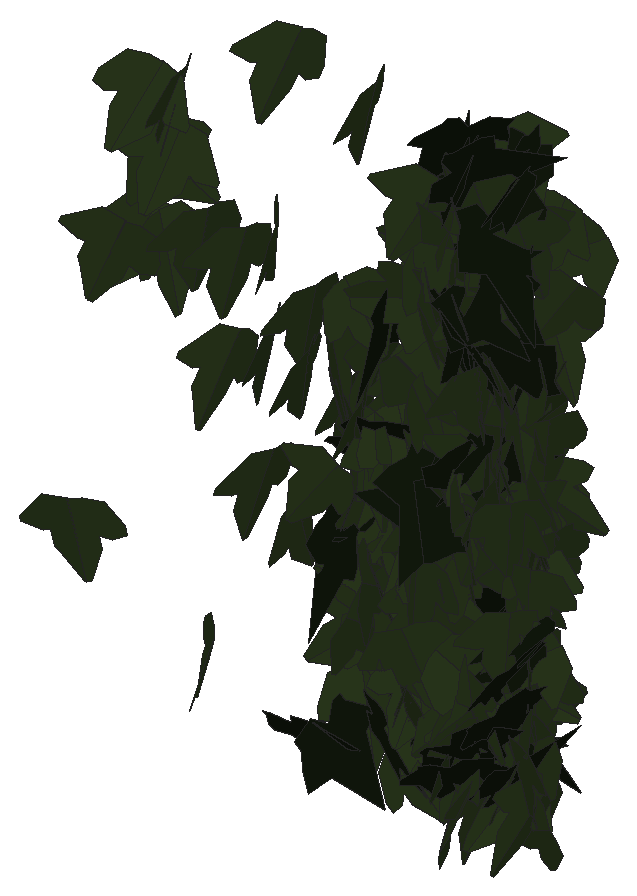
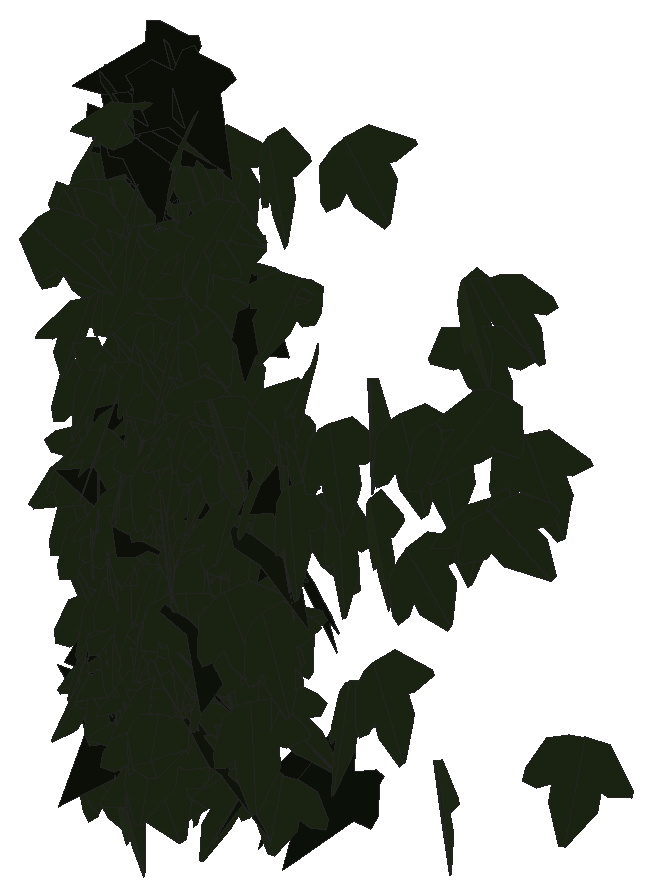
# SketchUp Ruby script. Lengths in inches.
U = 1.inch
M = Sketchup.active_model
def pt(a) = Geom::Point3d.new(a.map { |v| v * U })
def face(e, loops, mat)
  f = e.add_face(loops[0].map { |a| pt(a) })
  loops[1..].each { |l| e.add_face(l.map { |a| pt(a) }).erase! }
  f.material = f.back_material = mat if mat
  f
end
# faces: each face lists its corners as indices into pts; further lists are holes
def faces(e, pts, list, mat = nil) = list.each { |f| face(e, (f[0].is_a?(Array) ? f : [f]).map { |l| l.map { |i| pts[i] } }, mat) }
# xy, xz, yz: faces in a plane at the given z, y or x. An outline is a flat list of corners, or four numbers for a rectangle; further outlines are holes
def ring(l) = l.size == 4 ? [[l[0], l[1]], [l[2], l[1]], [l[2], l[3]], [l[0], l[3]]] : l.each_slice(2).to_a
def flat(e, list, mat, &to3) = list.each { |f| face(e, (f[0].is_a?(Array) ? f : [f]).map { |l| ring(l).map { |u, v| to3.(u, v) } }, mat) }
def xy(e, z, list, mat = nil) = flat(e, list, mat) { |x, y| [x, y, z] }
def xz(e, y, list, mat = nil) = flat(e, list, mat) { |x, z| [x, y, z] }
def yz(e, x, list, mat = nil) = flat(e, list, mat) { |y, z| [x, y, z] }
def lines(e, pts, list) = list.each { |a, b| e.add_line(pt(pts[a]), pt(pts[b])) }
# prism: a flat outline (further loops are holes) pulled along v
def prism(e, loops, v, mat = nil)
  f = face(e, loops, mat); d = Geom::Vector3d.new(v.map { |x| x * U })
  f.pushpull(f.normal.samedirection?(d) ? d.length : -d.length)
end
def box(e, o, s, mat = nil) = prism(e, [[o, [o[0] + s[0], o[1], o[2]], [o[0] + s[0], o[1] + s[1], o[2]], [o[0], o[1] + s[1], o[2]]]], [0, 0, s[2]], mat)
def at(x, y, z, deg = 0) = Geom::Transformation.translation(pt([x, y, z])) * Geom::Transformation.rotation(ORIGIN, Z_AXIS, deg.degrees)
def axes(o, x, y, z) = Geom::Transformation.new([*x, 0, *y, 0, *z, 0, *pt(o).to_a, 1])
def part(name) = M.definitions.add(name)
# library, detail: a bought-in or finely detailed component or shape, given as its bounding box
def library(name, o, s) = part(name).tap { |d| box(d.entities, o, s) }
def detail(e, o, s) = box(e.add_group.entities, o, s)
def put(e, d, t, mat = nil) = e.add_instance(d, t).tap { |i| i.material = mat if mat }
def group(e, t, mat = nil) = e.add_group.tap { |g| g.transformation = t; g.material = mat if mat }.entities
root = M.entities
M.materials.add("efeu1").color = [18, 25, 13]
M.materials.add("efeu2").color = [43, 57, 29]
c1 = part("ivyleaf_10")
p = [[0,0.5,-0.03],[-0.0625,2.02,-0.43],[-0.19,2.01,-0.46],[-0.54,1.05,-0.29],[-0.52,0.625,-0.18],[-0.83,0.76,-0.28],
  [-1.16,0.64,-0.33],[-1.15,0.33,-0.24],[-0.77,-0.39,0.02],[-0.3,-0.51,0.16],[0.04,-0.48,0.23],[-0.02,2.01,-0.4375],
  [-0.06,2.01,-0.43],[0.04,-0.49,0.23],[0.67,-0.49,0.14],[1.38,0.36,-0.2],[1.375,0.51,-0.24],[0.81,0.65,-0.19],
  [0.62,0.59,-0.15],[0.6,1.09,-0.28],[0.5,1.23,-0.31]]
faces(c1.entities,p,[[0,1,2,3,4,5,6,7,8,9,10],[11,12,0,13,14,15,16,17,18,19,20]],"efeu2")
c2 = part("ivyleaf_9")
p = [[1.54,2.16,1.25],[1.36,2.04,1.19],[-0.21,0.99,0.68],[-0.71,1.11,0.82],[-0.85,0.86,0.67],[-0.8,0.17,0.21],
  [-0.9,-0.01,0.1],[-0.67,-0.16,-0.02],[-0.08,-0.08,-0.05],[-0.03,-0.6,-0.4],[0.65,-0.88,-0.66],[0.83,-0.6,-0.49],
  [1.29,-0.42,-0.43],[1.8125,-0.07,-0.26],[1.21,0.44,0.15]]
faces(c2.entities,p,[[0,1,2,3,4,5,6,7,8,9,10,11,12,13,14]],"efeu1")
put(root,c1,axes([0.96,224.34,216.06],[-0.47039,-0.16713,-0.02836],[0.02619,0.01099,-0.49919],[0.16749,-0.47111,-0.00158]))
put(root,c1,axes([1.1875,225.43,219.52],[0.31206,0.2858,-0.26634],[-0.22229,-0.15043,-0.42185],[-0.32126,0.38169,0.03318]))
put(root,c1,axes([1.51,224.51,219.83],[-0.41225,-0.19131,0.20845],[-0.16107,-0.14417,-0.45086],[0.23261,-0.43888,0.05723]))
put(root,c1,axes([1.5,225.36,219.49],[0.05579,0.49599,0.02976],[-0.00377,0.03037,-0.49906],[-0.49686,0.05546,0.00713]))
put(root,c1,axes([1.57,225.19,220.67],[-0.1581,-0.36154,-0.30707],[0.26894,0.19831,-0.37195],[0.39074,-0.28278,0.13176]))
put(root,c1,axes([1.82,224.67,221.91],[0.46103,0.07291,-0.17927],[-0.17636,-0.03246,-0.46674],[-0.0797,0.49359,-0.00422]))
put(root,c1,axes([2.03,224.92,221.83],[0.1465,-0.47798,0.00877],[0.00356,-0.00808,-0.49992],[0.47804,0.14654,0.00103]))
put(root,c1,axes([2.11,224.74,221.18],[0.46588,0.12341,-0.13313],[-0.1388,0.00583,-0.48031],[-0.117,0.4845,0.03969]))
put(root,c1,axes([2.26,225.125,220],[-0.16365,-0.472,0.02088],[-0.00643,-0.01987,-0.49956],[0.47242,-0.16378,0.00044]))
put(root,c1,axes([2.54,225.25,218.39],[-0.09392,-0.42921,0.23866],[0.04424,-0.24939,-0.4311],[0.4891,-0.05986,0.08482]))
put(root,c1,axes([2.8,225.11,219.92],[-0.14469,-0.46928,0.09402],[0.00852,-0.10073,-0.48967],[0.47853,-0.1401,0.03714]))
put(root,c1,axes([2.88,225.47,216.86],[-0.04373,-0.49068,0.08555],[0.00052,-0.08593,-0.49256],[0.49808,-0.04299,0.00802]))
put(root,c1,axes([3,224.25,215.01],[0.21326,-0.39005,-0.22888],[-0.0988,0.20675,-0.4444],[0.44132,0.23477,0.01111]))
put(root,c1,axes([3.13,225.24,218.76],[0.17755,-0.46436,-0.05333],[-0.00564,0.05491,-0.49694],[0.46738,0.17706,0.01426]))
put(root,c1,axes([3.26,225.14,220.21],[0.19492,-0.39777,-0.23192],[-0.05057,0.23182,-0.44011],[0.45766,0.19503,0.05014]))
put(root,c1,axes([3.33,225.48,216.4375],[0.09135,-0.45267,-0.1917],[0.0624,0.20408,-0.45217],[0.48761,0.05869,0.09378]))
put(root,c1,axes([3.6,225.28,218.55],[0.07334,-0.47095,-0.15108],[-0.02799,0.14853,-0.47661],[0.4938,0.07837,-0.00458]))
put(root,c1,axes([3.77,225.21,219.48],[-0.06818,-0.49522,-0.01044],[0.00123,0.01037,-0.49989],[0.49533,-0.06819,-0.00019]))
put(root,c1,axes([3.8,224.81,223.01],[-0.21603,-0.39611,0.21548],[-0.0125,-0.23357,-0.44191],[0.45075,-0.19632,0.09101]))
put(root,c1,axes([4.31,225.27,218.5],[0.0717,-0.48644,-0.09072],[0.00628,0.09256,-0.49132],[0.49479,0.06932,0.01938]))
put(root,c1,axes([4.5,225.4375,216.91],[-0.03153,-0.49581,0.05635],[-0.00224,-0.05632,-0.49681],[0.499,-0.03159,0.00133]))
put(root,c1,axes([4.71,224.38,217.85],[-0.36088,-0.07697,0.27837],[-0.2598,-0.13092,-0.35148],[0.15159,-0.40763,0.06032]))
put(root,c2,axes([4.4,224.12,214.57],[0.43898,0.13994,-0.06919],[-0.09411,0.05199,-0.43992],[-0.13838,0.40858,0.07967]))
put(root,c1,axes([4.8125,224.95,215.67],[0.34304,-0.0201,-0.3632],[-0.36196,0.03072,-0.34357],[0.03613,0.49865,0.00653]))
put(root,c1,axes([4.66,225.55,215.74],[-0.16669,-0.47025,-0.03289],[0.00787,0.03211,-0.49891],[0.47133,-0.16685,-0.0033]))
put(root,c1,axes([4.87,224.73,217.83],[0.19361,-0.39179,-0.24293],[-0.11098,0.21612,-0.43701],[0.44743,0.22314,-0.00327]))
put(root,c1,axes([4.61,225.07,214.73],[0.46794,0.10225,0.14346],[0.13534,0.05202,-0.47852],[-0.11279,0.48666,0.02101]))
put(root,c1,axes([4.94,225.1875,216.31],[-0.47803,-0.05598,0.13549],[-0.13614,-0.00191,-0.4811],[0.05438,-0.49685,-0.01342]))
put(root,c1,axes([4.78,224.46,218.87],[-0.34673,0.29272,-0.02245],[0.00861,-0.02329,-0.45168],[-0.31688,-0.32093,0.0123]))
put(root,c1,axes([4.86,224.91,222.66],[0.10278,-0.48698,-0.04785],[-0.00495,0.04785,-0.49768],[0.4893,0.10278,0.00502]))
put(root,c2,axes([4.87,224.38,217.11],[-0.37707,0.05574,-0.26356],[0.27267,-0.02508,-0.36748],[-0.06468,-0.43068,-0.01271]))
put(root,c1,axes([4.83,224.33,219.67],[-0.15891,0.40661,-0.04926],[0.00632,-0.04824,-0.44957],[-0.44206,-0.14685,0.01128]))
put(root,c2,axes([5.2,224.65,217.49],[-0.13651,0.37995,0.17676],[-0.17867,0.11713,-0.40028],[-0.4125,-0.17647,0.11488]))
put(root,c1,axes([5.0625,225.41,216.97],[-0.20223,-0.4241,0.17101],[-0.00333,-0.18562,-0.46426],[0.45727,-0.18891,0.07225]))
put(root,c2,axes([4.9,224.15,214.7],[0.10876,-0.25337,-0.35251],[-0.14432,0.31155,-0.28349],[0.43365,0.16723,-0.00594]))
put(root,c1,axes([4.97,225,219.26],[0.0369,-0.36666,0.33793],[0.12839,-0.32044,-0.36171],[0.48182,0.11347,0.0705]))
put(root,c1,axes([5.08,224.52,218.6],[-0.43364,0.16052,-0.04923],[-0.02147,-0.16793,-0.41682],[-0.17946,-0.36777,0.16883]))
put(root,c1,axes([5.17,224.33,218.92],[0.0818,-0.37126,-0.22221],[-0.04888,0.20883,-0.39406],[0.46003,0.0882,-0.00236]))
put(root,c1,axes([4.83,225.12,216.41],[0.35816,-0.09659,0.33525],[0.32701,-0.07452,-0.37083],[0.1216,0.48489,0.00979]))
put(root,c1,axes([5.4,224.52,216.24],[0.1932,0.12468,0.39146],[-0.34982,-0.19223,0.22632],[0.247,-0.36977,0.01434]))
put(root,c1,axes([5.04,225.17,216.64],[-0.44515,0.05357,-0.22129],[0.21516,-0.05996,-0.44734],[-0.07447,-0.49349,0.03033]))
put(root,c1,axes([5.26,224.81,217.61],[-0.2177,-0.44259,-0.082],[0.04095,0.07124,-0.4932],[0.44825,-0.22146,0.00523]))
put(root,c1,axes([5.33,224.4375,216.76],[-0.3028,0.27586,0.19322],[-0.14349,0.12987,-0.40906],[-0.32929,-0.31026,0.00057]))
put(root,c2,axes([5.02,224.45,218.44],[0.40584,0.12435,0.18764],[0.17225,0.09041,-0.41026],[-0.16229,0.40692,0.03381]))
put(root,c1,axes([5.24,224.19,216.22],[-0.07236,-0.29876,-0.39434],[0.12552,0.37441,-0.30669],[0.47855,-0.14338,0.02082]))
put(root,c1,axes([5.24,225.3,218.19],[-0.02706,0.49926,0.00329],[-0.00013,0.00329,-0.49999],[-0.49927,-0.02706,-0.00005]))
put(root,c1,axes([5.17,224.74,218.29],[-0.01169,-0.46038,0.19472],[0.25019,-0.17402,-0.39639],[0.43275,0.08816,0.23443]))
put(root,c1,axes([5.22,224.17,220.49],[0.21395,0.33695,0.19854],[0.03353,0.19993,-0.40049],[-0.41691,0.18899,0.06968]))
put(root,c1,axes([5.3,225.09,218.53],[0.31704,-0.38619,0.01861],[0.00301,0.02653,0.49929],[-0.38663,-0.31647,0.01915]))
put(root,c1,axes([5.4375,224.11,216.8],[0.16934,-0.22854,-0.41121],[-0.00934,0.43532,-0.24579],[0.47036,0.09092,0.14316]))
put(root,c2,axes([5.31,224.47,214.8],[0.372,-0.13798,-0.23611],[-0.21395,0.11429,-0.38483],[0.19118,0.39639,0.02876]))
put(root,c1,axes([5.47,225.1875,218.97],[-0.19538,-0.45916,0.03151],[0.03111,-0.04733,-0.49678],[0.45919,-0.19217,0.04707]))
put(root,c2,axes([5.7,225.125,215.02],[-0.35311,0.28481,0.03615],[-0.03083,0.02015,-0.45094],[-0.30834,-0.32818,0.00369]))
put(root,c1,axes([5.5,225.19,219.11],[-0.25973,-0.42384,0.05387],[0.01978,-0.0749,-0.49396],[0.42679,-0.25446,0.05567]))
put(root,c1,axes([5.5,225.07,216.81],[-0.49206,0.07211,-0.05173],[0.05092,-0.00934,-0.49731],[-0.07269,-0.49468,0.00185]))
put(root,c2,axes([5.625,224.55,217.23],[0.2706,0.05186,-0.36586],[-0.38344,0.01246,-0.26107],[-0.02144,0.43172,0.05148]))
put(root,c1,axes([5.65,224.76,215.72],[0.34046,-0.21633,-0.29544],[-0.19484,0.23454,-0.39627],[0.31004,0.38496,0.0754]))
put(root,c1,axes([5.52,225.2,219.25],[0.38803,0.30743,-0.07012],[-0.09449,0.0073,-0.49094],[-0.30083,0.39425,0.06377]))
put(root,c1,axes([5.6,224.78,215.54],[0.26224,-0.41911,-0.07469],[-0.05121,0.05604,-0.4942],[0.42262,0.26685,-0.01353]))
put(root,c2,axes([5.5,224.55,220.36],[-0.12922,0.11287,-0.41881],[0.32083,-0.2719,-0.17105],[-0.31794,-0.32024,-0.00238]))
put(root,c1,axes([5.57,224.97,218.71],[-0.092,0.41612,0.26149],[-0.06876,0.25252,-0.42604],[-0.48663,-0.11435,0.01076]))
put(root,c1,axes([5.72,224.52,215.29],[-0.39409,0.21502,0.22013],[-0.186,0.11851,-0.44873],[-0.24515,-0.43557,-0.01342]))
put(root,c2,axes([5.69,224.84,216.53],[0.0985,0.41342,0.10395],[-0.0361,0.10888,-0.43662],[-0.45794,0.08034,0.05678]))
put(root,c1,axes([5.48,224.67,217.5],[0.40548,0.20234,0.08901],[0.04293,0.1041,-0.4373],[-0.23335,0.37074,0.07422]))
put(root,c1,axes([5.51,224.72,214.23],[0.05243,0.37583,0.22213],[0.02649,0.21219,-0.3941],[-0.46611,0.05433,0.00259]))
put(root,c1,axes([5.59,224.74,216.61],[0.15025,-0.36342,0.20219],[-0.07728,0.18077,0.4047],[-0.43836,-0.15643,-0.00205]))
put(root,c1,axes([5.48,225.2,218.95],[0.37773,0.3164,0.08491],[0.06534,0.05422,-0.49274],[-0.32101,0.38334,-0.00039]))
put(root,c1,axes([5.97,224.43,220.58],[0.06268,0.07088,-0.49097],[-0.49044,-0.06542,-0.07206],[-0.07445,0.49061,0.06132]))
put(root,c1,axes([5.73,224.95,217.1],[-0.28725,-0.38413,0.1412],[-0.03193,-0.15094,-0.4756],[0.40801,-0.28225,0.06218]))
put(root,c1,axes([5.51,224.68,218.66],[0.33555,0.35656,0.10137],[0.06464,0.07836,-0.48957],[-0.36501,0.34165,0.00649]))
put(root,c1,axes([5.7,224.96,215.88],[-0.17881,0.39512,0.24881],[-0.12381,0.21678,-0.43322],[-0.45022,-0.21654,0.02031]))
put(root,c1,axes([5.54,225.19,219.35],[-0.18036,-0.2456,-0.39643],[0.24359,0.31283,-0.30463],[0.39766,-0.30302,0.0068]))
put(root,c1,axes([5.6875,224.78,215.35],[0.44084,0.12069,-0.09327],[-0.09447,-0.02042,-0.44265],[-0.13208,0.41742,0.00531]))
put(root,c1,axes([5.4375,224.53,217.4],[0.35522,-0.05698,0.29008],[0.2945,-0.05938,-0.34703],[0.08833,0.42714,-0.00954]))
put(root,c1,axes([5.64,224.9,221.64],[0.01604,0.38669,0.20664],[0.01691,0.1982,-0.40238],[-0.46922,0.02036,-0.00743]))
put(root,c1,axes([5.8,225.32,216.65],[-0.42548,-0.25136,0.07605],[-0.01045,-0.12848,-0.4831],[0.2624,-0.41269,0.10408]))
put(root,c1,axes([6.08,224.88,215.33],[-0.00949,0.01786,-0.45193],[-0.46934,0.01679,0.00985],[0.01853,0.43431,0.0182]))
put(root,c1,axes([5.85,224.6875,216.83],[-0.40801,-0.28893,-0.00655],[0.00639,0.00232,-0.49995],[0.28894,-0.40806,0.0018]))
put(root,c1,axes([5.61,224.91,214.64],[0.31094,0.27164,0.28201],[0.18685,0.21352,-0.4117],[-0.34409,0.36142,0.03128]))
put(root,c1,axes([5.93,224.7,216.53],[0.22916,0.33461,-0.29244],[-0.22019,-0.2003,-0.40174],[-0.38601,0.31291,0.05555]))
put(root,c1,axes([5.92,225.12,219.34],[0.01265,-0.49976,0.00899],[-0.00138,-0.00903,-0.49992],[0.49984,0.01263,-0.00161]))
put(root,c1,axes([6.11,224.84,217.27],[-0.21808,-0.22314,0.3907],[-0.14851,-0.37415,-0.29658],[0.42472,-0.2454,0.09691]))
put(root,c1,axes([6.08,224.33,217.13],[-0.48049,0.06173,0.12376],[-0.12947,-0.04341,-0.48099],[-0.04864,-0.49427,0.0577]))
put(root,c1,axes([6.15,224.42,222.05],[-0.36892,-0.22702,0.24972],[-0.16361,-0.20328,-0.42651],[0.29518,-0.39641,0.0757]))
put(root,c1,axes([6.3,224.32,221.45],[0.128,-0.04012,-0.48167],[-0.44171,0.19259,-0.13342],[0.19624,0.45967,0.01386]))
put(root,c1,axes([5.76,225.08,220.26],[-0.38216,-0.03717,-0.32027],[0.31642,-0.13863,-0.36147],[-0.06193,-0.47896,0.12949]))
put(root,c2,axes([6.24,225.05,215.9],[-0.44758,0.12759,0.03602],[-0.03986,-0.00222,-0.45076],[-0.13711,-0.41586,0.01346]))
put(root,c1,axes([5.95,224.29,216.125],[-0.39357,-0.2733,-0.14287],[0.1335,0.05782,-0.47837],[0.27799,-0.41469,0.02746]))
put(root,c1,axes([6,224.9,216.33],[-0.11789,-0.46707,-0.13396],[0.06542,0.12133,-0.48062],[0.48148,-0.13085,0.03251]))
put(root,c1,axes([5.8125,224.53,219.58],[-0.3724,-0.09127,-0.32092],[0.31974,0.03979,-0.38234],[0.09533,-0.48999,0.02873]))
put(root,c1,axes([6.02,224.7,217.61],[-0.26171,-0.41365,-0.10197],[0.09865,0.05758,-0.48678],[0.41446,-0.27491,0.05147]))
put(root,c1,axes([6.02,224.42,219.27],[-0.08478,0.40206,0.15216],[-0.04841,0.14021,-0.42571],[-0.45954,-0.08894,0.01678]))
put(root,c1,axes([5.9,225,216.51],[-0.21044,-0.30521,-0.3355],[0.25088,0.22979,-0.36641],[0.37785,-0.32256,0.05642]))
put(root,c1,axes([6.1,225.04,219.91],[0.05733,-0.27977,-0.41042],[-0.03033,0.4104,-0.284],[0.49578,0.05746,0.03009]))
put(root,c1,axes([6.04,225.54,214.61],[0.32985,0.3541,-0.12574],[-0.10522,-0.07357,-0.48323],[-0.36073,0.34525,0.02598]))
put(root,c1,axes([5.99,224.58,221.01],[0.0547,0.4839,0.11337],[-0.01367,0.11548,-0.48629],[-0.49681,0.05011,0.02586]))
put(root,c1,axes([6.08,225.55,215.08],[-0.33177,-0.36629,-0.07592],[0.0608,0.04732,-0.49403],[0.3691,-0.33704,0.01314]))
put(root,c1,axes([6.05,224.6,220.87],[-0.22059,0.44864,-0.0076],[0.00313,-0.00693,-0.49994],[-0.4487,-0.22062,0.00025]))
put(root,c1,axes([6.2,224.5625,221.79],[0.33609,-0.31942,-0.18712],[-0.1379,0.12652,-0.46365],[0.34355,0.36327,-0.00305]))
put(root,c1,axes([5.97,225.15,221.18],[-0.38275,0.06707,-0.25289],[0.24936,-0.08259,-0.37367],[-0.10969,-0.42179,0.03296]))
put(root,c1,axes([6.04,224.97,221.13],[0.46682,0.17604,0.03307],[0.02925,0.01617,-0.49888],[-0.17671,0.46771,0.0048]))
put(root,c1,axes([6.1875,225.22,217.83],[0.25401,-0.40204,-0.1544],[-0.03891,0.15709,-0.47308],[0.42891,0.25235,0.04852]))
put(root,c1,axes([6.17,224.74,218.03],[-0.15367,-0.43519,-0.19234],[0.08152,0.17505,-0.46121],[0.46876,-0.17311,0.01715]))
put(root,c1,axes([6.4375,224.75,218.6],[0.29107,-0.05559,-0.40272],[-0.39439,0.08158,-0.29631],[0.09865,0.49016,0.00364]))
put(root,c1,axes([6.15,224.66,218.05],[-0.45059,0.20546,-0.06897],[0.06166,-0.03101,-0.49521],[-0.20777,-0.45478,0.00261]))
put(root,c2,axes([6.22,224.57,218.1875],[-0.25707,-0.36345,0.02252],[-0.01784,-0.01507,-0.4518],[0.39282,-0.23854,-0.00578]))
put(root,c1,axes([6.29,224.19,220.58],[-0.23098,0.33112,0.19131],[-0.09786,0.16039,-0.40983],[-0.39722,-0.23207,-0.01028]))
put(root,c2,axes([6.63,224.29,218],[-0.2798,0.08447,0.35264],[-0.35104,0.09672,-0.28334],[-0.13856,-0.41561,0.00574]))
put(root,c1,axes([6.26,225.22,216.73],[0.05282,-0.42368,-0.26021],[0.06473,0.2653,-0.41884],[0.49297,0.01056,0.08288]))
put(root,c1,axes([6.43,225.41,216.06],[-0.25662,-0.3441,0.25641],[-0.12968,-0.22261,-0.42852],[0.40906,-0.28643,0.02501]))
put(root,c1,axes([6.23,225.44,215.59],[-0.05426,0.48926,-0.08761],[0.00008,-0.08812,-0.49217],[-0.49705,-0.05343,0.00948]))
put(root,c1,axes([6.36,225.01,218.41],[-0.49906,-0.03048,-0.00342],[0.00342,0.00018,-0.49999],[0.03048,-0.49907,0.00003]))
put(root,c2,axes([6.49,224.35,220.68],[0.19912,0.0071,-0.40969],[-0.42535,0.01541,-0.19141],[0.01183,0.43467,0.01348]))
put(root,c1,axes([6.38,225.125,218.14],[-0.03024,-0.49038,0.09281],[-0.01067,-0.09232,-0.49129],[0.49897,-0.0317,-0.00488]))
put(root,c1,axes([6.27,224.52,215.875],[0.47837,-0.14478,0.01424],[0.01433,-0.00183,-0.49979],[0.14477,0.47858,0.0024]))
put(root,c1,axes([6.6,224.5,215.32],[-0.29415,-0.15165,0.31553],[-0.26778,-0.17649,-0.32324],[0.24996,-0.36753,0.02503]))
put(root,c1,axes([6.14,225.28,219.46],[0.41092,0.10785,0.18842],[0.18615,0.0562,-0.41124],[-0.13116,0.41765,0.00668]))
put(root,c1,axes([6.34,225.56,219.81],[-0.03044,0.28892,-0.33693],[-0.0494,-0.32482,-0.29712],[-0.4662,0.01556,0.05348]))
put(root,c1,axes([6.02,224.7,216.54],[-0.01821,-0.03774,-0.45035],[0.42686,-0.18169,0.00047],[-0.19538,-0.39343,0.04299]))
put(root,c1,axes([6.3125,225.43,215.75],[0.01704,0.49893,-0.02782],[-0.001,-0.0278,-0.49923],[-0.49971,0.01707,0.00005]))
put(root,c1,axes([6.35,225.11,219.87],[-0.48421,-0.04987,-0.11427],[0.11336,0.0147,-0.48676],[0.05191,-0.49729,-0.00293]))
put(root,c2,axes([6.57,224.55,222.98],[-0.02308,0.33714,-0.28502],[-0.0752,-0.2735,-0.34427],[-0.46317,0.02761,0.07009]))
put(root,c1,axes([6.46,224.43,214.82],[0.04985,-0.32835,-0.29283],[-0.0328,0.28001,-0.34477],[0.466,0.05483,0.00706]))
put(root,c1,axes([6.39,225.39,216.05],[0.00414,-0.36996,0.33633],[0.07106,-0.33249,-0.36661],[0.49491,0.05084,0.04982]))
put(root,c1,axes([6.36,224.73,217.35],[-0.29286,0.33239,-0.07507],[0.03464,-0.06692,-0.44577],[-0.36572,-0.27251,0.0179]))
put(root,c2,axes([6.74,224.28,220.48],[-0.16708,0.05128,-0.41945],[-0.41412,0.12504,0.1695],[0.14595,0.41347,0.00076]))
put(root,c1,axes([6.59,224.18,213.81],[0.1938,-0.07073,0.4055],[-0.26915,0.31263,0.17826],[-0.33273,-0.29409,0.09198]))
put(root,c1,axes([6.7,224.6,219.42],[-0.17281,0.15753,0.38747],[-0.35365,0.18478,-0.22752],[-0.25648,-0.36092,0.05264]))
put(root,c1,axes([6.45,224.46,222.3125],[-0.26188,0.41893,0.07694],[-0.02731,0.07362,-0.4938],[-0.42506,-0.26283,-0.01568]))
put(root,c1,axes([6.37,224.6,215.5625],[0.46744,0.02895,0.03387],[0.03512,0.00169,-0.45113],[-0.03132,0.43403,-0.00051]))
put(root,c1,axes([6.6,225.39,215.27],[-0.40215,-0.23111,0.18671],[-0.06919,-0.23273,-0.43709],[0.28894,-0.37739,0.15521]))
put(root,c1,axes([6.57,225.33,216.71],[-0.14812,-0.47163,-0.075],[0.00986,0.07549,-0.49417],[0.47746,-0.14787,-0.01306]))
put(root,c1,axes([6.56,225.41,215.97],[0.0901,-0.48687,-0.0696],[-0.00033,0.0707,-0.49498],[0.49182,0.08924,0.01241]))
put(root,c1,axes([6.2,225.5,219.47],[0.15564,-0.09005,-0.41645],[0.3593,-0.22292,0.17665],[-0.2596,-0.36252,-0.00518]))
put(root,c1,axes([6.42,225.22,214.9375],[0.26398,0.3516,0.0796],[0.04482,0.06437,-0.44533],[-0.38603,0.24791,0.00273]))
put(root,c1,axes([6.51,224.51,217.86],[-0.48026,-0.09122,-0.10501],[0.10389,0.01575,-0.48883],[0.09249,-0.49136,0.00382]))
put(root,c1,axes([6.54,224.51,214.72],[0.41764,-0.19212,-0.05481],[-0.04331,0.03766,-0.44877],[0.21075,0.38846,0.01639]))
put(root,c1,axes([6.5625,225.53,214.99],[0.31436,-0.36449,-0.13536],[-0.01584,0.16191,-0.47279],[0.38849,0.30154,0.09025]))
put(root,c1,axes([6.51,224.37,218.09],[-0.45345,0.05909,-0.10112],[0.10439,-0.01089,-0.44095],[-0.06483,-0.43083,-0.00272]))
put(root,c1,axes([6.7,224.23,221.06],[-0.19109,0.2088,0.35164],[-0.23468,0.25905,-0.28463],[-0.35933,-0.28022,-0.00111]))
put(root,c2,axes([6.68,224.125,214.78],[0.19428,0.38235,-0.10744],[-0.11951,-0.06042,-0.43298],[-0.41071,0.19845,0.07517]))
put(root,c1,axes([6.81,224.4,218.77],[-0.39679,-0.1049,0.21626],[-0.20465,-0.09117,-0.39603],[0.14625,-0.4122,0.03256]))
put(root,c1,axes([6.24,225.47,215.62],[0.17479,0.08336,0.46098],[0.42028,0.18942,-0.19361],[-0.20691,0.45516,-0.00385]))
put(root,c1,axes([6.6,225.18,215.08],[0.44638,-0.12795,-0.04679],[-0.04396,0.02063,-0.4499],[0.13973,0.41525,0.00793]))
put(root,c2,axes([6.3,224.86,214.35],[0.27679,0.30817,-0.1758],[0.11974,0.12764,0.41683],[0.36023,-0.27922,-0.00348]))
put(root,c1,axes([6.64,225.36,214.1],[0.20635,-0.45525,0.01295],[0.00548,-0.01174,-0.49983],[0.4554,0.20642,0.00015]))
put(root,c2,axes([6.79,224.05,222.39],[0.03496,0.12379,0.43239],[-0.04189,0.41607,-0.1257],[-0.46662,-0.02808,0.04368]))
put(root,c1,axes([6.71,225.37,216.41],[-0.09666,-0.48883,-0.04131],[0.00402,0.04132,-0.49827],[0.49055,-0.09666,-0.00406]))
put(root,c2,axes([6.93,225.11,214.84],[-0.41231,0.20796,0.01564],[-0.03572,-0.02941,-0.45005],[-0.22234,-0.38093,0.04329]))
put(root,c1,axes([6.67,224.94,221.46],[0.04725,-0.43241,-0.24656],[0.0523,0.25061,-0.42949],[0.49501,0.01479,0.06891]))
put(root,c1,axes([6.49,224.68,217.17],[-0.06643,-0.29703,-0.39669],[0.293,0.29925,-0.27313],[0.39967,-0.26875,0.13431]))
put(root,c2,axes([6.8125,224.4,219.86],[0.05252,-0.18141,0.40806],[-0.04356,0.39121,0.19331],[-0.46482,-0.05716,0.02799]))
put(root,c1,axes([6.9,224.73,219.67],[-0.34534,0.13349,0.2735],[-0.27239,0.07729,-0.35973],[-0.1651,-0.40673,0.02141]))
put(root,c2,axes([7.07,224.64,221.11],[-0.25795,0.13822,0.34971],[-0.31221,0.17179,-0.28699],[-0.23812,-0.37498,-0.00257]))
put(root,c1,axes([6.51,224.34,216.01],[0.16505,0.26308,0.32333],[0.13547,0.28552,-0.3154],[-0.41847,0.19619,0.02542]))
put(root,c1,axes([6.625,224.98,215.99],[0.25083,0.36775,-0.00678],[-0.02374,0.00618,-0.45178],[-0.39653,0.23226,0.02275]))
put(root,c1,axes([6.67,225.34,216.82],[0.04771,0.32047,0.38082],[-0.06814,0.38317,-0.31391],[-0.49303,-0.02195,0.08024]))
put(root,c1,axes([6.77,224.64,215.09],[-0.11817,-0.47796,0.08712],[-0.02286,-0.08409,-0.49235],[0.4853,-0.12035,-0.00197]))
put(root,c1,axes([6.72,224.74,214.31],[0.06242,-0.48592,0.0999],[0.02336,-0.0977,-0.48981],[0.49554,0.06582,0.01051]))
put(root,c2,axes([6.92,224.89,216.74],[-0.21709,0.38576,-0.00325],[-0.00047,-0.00375,-0.45238],[-0.41663,-0.201,0.0022]))
put(root,c1,axes([6.79,225.27,217.36],[0.32411,0.26169,-0.27653],[-0.225,-0.1613,-0.41636],[-0.30712,0.39434,0.0132]))
put(root,c2,axes([7.06,224.67,219.0625],[-0.0996,0.00832,-0.44203],[-0.45113,-0.08254,0.09258],[-0.08526,0.42702,0.0265]))
put(root,c2,axes([6.77,225.02,215.85],[0.27688,0.3182,-0.15511],[-0.10432,-0.11369,-0.42496],[-0.36492,0.27394,0.0038]))
put(root,c1,axes([6.81,224.95,220.3],[-0.28051,-0.40981,0.05802],[-0.00956,-0.06365,-0.49584],[0.41379,-0.27929,0.02788]))
put(root,c1,axes([6.68,224.4,218.32],[-0.0639,0.42805,-0.05193],[0.00087,-0.05029,-0.44937],[-0.46543,-0.05887,0.00629]))
put(root,c1,axes([6.78,225.26,217.4375],[-0.03369,-0.49061,-0.09037],[0.0078,0.09004,-0.49176],[0.4988,-0.03454,0.00158]))
put(root,c1,axes([7.07,224.47,219.66],[-0.17517,0.07152,-0.41313],[-0.38728,0.17099,0.18429],[0.2001,0.39354,-0.00499]))
put(root,c1,axes([6.93,224.43,217.88],[-0.41996,-0.10421,0.1714],[-0.1649,-0.06593,-0.41803],[0.13097,-0.41716,0.02326]))
put(root,c2,axes([6.89,224.72,222.43],[-0.00033,0.42303,-0.10541],[0.00376,-0.10135,-0.43994],[-0.46978,-0.00111,-0.00345]))
put(root,c2,axes([7.04,224.55,219.26],[-0.16511,0.31277,0.27126],[-0.11135,0.2398,-0.3619],[-0.42551,-0.18411,-0.01055]))
put(root,c2,axes([6.7,224.16,215.08],[0.29638,0.3262,0.09013],[0.05832,0.06782,-0.44333],[-0.35982,0.27967,0.00238]))
put(root,c2,axes([7.15,224.98,222.22],[-0.3355,0.04299,0.31351],[-0.32484,0.02379,-0.32589],[-0.05124,-0.43222,0.01324]))
put(root,c2,axes([6.51,224.34,220.67],[0.33722,-0.30001,0.04317],[0.03226,-0.02883,-0.45034],[0.3255,0.31367,-0.00009]))
put(root,c1,axes([6.59,224.52,215.6],[-0.29939,0.18303,-0.29209],[0.25948,-0.14568,-0.34536],[-0.25248,-0.36675,-0.00859]))
put(root,c2,axes([6.68,224.77,216.72],[0.3746,0.26125,0.02679],[0.02455,0.01263,-0.45159],[-0.28246,0.34758,-0.00372]))
put(root,c1,axes([6.76,224.97,220.82],[-0.28309,-0.36875,-0.18407],[0.13748,0.12603,-0.46392],[0.38854,-0.31327,0.03004]))
put(root,c2,axes([6.52,224.35,218.33],[0.16024,0.03778,0.42345],[0.40126,0.16847,-0.15706],[-0.18447,0.39927,0.02621]))
put(root,c1,axes([7.125,224.37,220.71],[-0.21767,-0.08498,0.39105],[-0.36507,-0.16501,-0.22722],[0.20013,-0.39342,0.01083]))
put(root,c2,axes([7.06,224.37,219.22],[-0.32938,0.31003,0.00985],[-0.00758,0.00639,-0.45229],[-0.33491,-0.30506,0.00054]))
put(root,c1,axes([6.82,225.15,215.08],[0.491,-0.0574,-0.07497],[-0.07321,0.01927,-0.49424],[0.05962,0.49632,0.01052]))
put(root,c1,axes([6.91,224.61,218.86],[-0.33422,0.26399,0.16033],[-0.13125,0.09506,-0.42299],[-0.30296,-0.33241,0.00637]))
put(root,c1,axes([6.9375,224.45,218.9],[0.15324,-0.17436,-0.44285],[-0.10549,0.44122,-0.21022],[0.4641,0.15786,0.09844]))
put(root,c1,axes([6.77,224.61,218.53],[0.21668,0.38586,-0.00968],[-0.00468,-0.00823,-0.4523],[-0.41682,0.20068,0.00005]))
put(root,c2,axes([6.68,225.15,214.91],[0.45831,0.09494,-0.01169],[-0.0122,-0.00098,-0.45225],[-0.10253,0.42451,0.00157]))
put(root,c1,axes([6.81,224.95,215.24],[0.07448,0.42941,0.00904],[-0.0012,0.00898,-0.4523],[-0.46386,0.06893,0.00263]))
put(root,c1,axes([6.97,224.95,214.26],[0.29237,0.22415,-0.26657],[-0.21336,-0.16331,-0.36552],[-0.29952,0.33513,0.00017]))
put(root,c1,axes([6.92,224.32,219.92],[-0.15715,-0.46333,-0.10307],[0.03687,0.09633,-0.48924],[0.47323,-0.16137,0.00389]))
put(root,c1,axes([6.79,225.16,222.64],[0.15802,0.39354,0.11833],[0.05374,0.10285,-0.43652],[-0.43915,0.1542,-0.01084]))
put(root,c1,axes([6.84,225.01,215.8],[0.11359,0.42197,0.01055],[0.00056,0.01033,-0.45227],[-0.45586,0.10516,0.00208]))
put(root,c1,axes([7.01,225.39,221.59],[-0.39806,-0.22578,0.05099],[-0.05048,-0.01753,-0.44941],[0.24436,-0.37141,-0.00978]))
put(root,c1,axes([6.9,224.34,222.43],[-0.35274,-0.26427,-0.11725],[0.09958,0.06526,-0.43688],[0.29389,-0.3393,0.0073]))
put(root,c1,axes([7.11,225.16,214.8],[-0.03742,-0.03718,-0.4493],[-0.30447,-0.32737,0.05282],[-0.35582,0.28403,0.00206]))
put(root,c1,axes([6.59,225.15,214.55],[0.26059,-0.14463,0.40146],[0.41032,-0.04424,-0.28228],[0.11718,0.47657,0.09563]))
put(root,c2,axes([6.8,224.82,217.49],[-0.03486,0.4118,-0.14184],[-0.01374,0.13581,0.42958],[0.4683,0.03464,0.00204]))
put(root,c1,axes([7.08,225.1,217.58],[-0.32267,0.20702,0.24852],[-0.20826,0.14123,-0.37799],[-0.2706,-0.35556,-0.00544]))
put(root,c2,axes([7.1,224.75,215.54],[-0.15421,0.40395,-0.07826],[0.03364,-0.0688,-0.44553],[-0.44249,-0.146,-0.00659]))
put(root,c1,axes([6.97,224.87,221.6],[0.08474,-0.4857,0.08316],[-0.00057,-0.08448,-0.49281],[0.49277,0.08343,-0.01487]))
put(root,c2,axes([7.08,224.86,222.32],[-0.2233,0.3365,-0.18961],[0.10885,-0.15204,-0.4107],[-0.39875,-0.22995,-0.00593]))
put(root,c1,axes([7.07,224.51,219.47],[0.28226,-0.27896,-0.21592],[-0.15243,0.15227,-0.39755],[0.34323,0.29702,0.00101]))
put(root,c1,axes([6.91,225.22,217.75],[-0.05847,0.49559,-0.03123],[0.00137,-0.03128,-0.49902],[-0.49657,-0.05845,0.0023]))
put(root,c1,axes([7.07,225.24,217.2],[-0.27216,-0.41726,0.04273],[-0.02013,-0.03789,-0.49816],[0.41896,-0.27287,0.00382]))
put(root,c1,axes([7.03,224.5,218.44],[0.03983,-0.44678,-0.22091],[0.00133,0.22171,-0.44815],[0.49841,0.03511,0.01885]))
put(root,c1,axes([7.0625,225.07,217.79],[-0.33678,0.28123,0.1181],[-0.08631,0.08093,-0.43666],[-0.31598,-0.32185,-0.0066]))
put(root,c1,axes([7.02,225.31,217.11],[0.30723,-0.37784,-0.11334],[0.00462,0.1471,-0.47785],[0.39445,0.29257,0.09388]))
put(root,c2,axes([7.29,224.84,216.39],[-0.43191,0.16986,0.02174],[-0.04967,-0.05548,-0.44615],[-0.17804,-0.3966,0.07172]))
put(root,c1,axes([7.11,225.06,216.92],[-0.4419,0.12444,0.0827],[-0.0808,0.02725,-0.44476],[-0.1375,-0.41593,-0.0044]))
put(root,c1,axes([6.96,224.53,221.45],[0.07564,0.42855,-0.02681],[-0.00667,-0.02511,-0.4516],[-0.46362,0.07028,0.00213]))
put(root,c2,axes([6.85,224.03,222.74],[0.0461,0.24294,-0.37264],[0.04993,0.35543,0.25635],[0.46486,-0.06227,0.00941]))
put(root,c1,axes([7.09,225.26,217.73],[0.22207,-0.40147,-0.19875],[0.00011,0.22188,-0.44807],[0.44798,0.19896,0.09863]))
put(root,c1,axes([7.3125,224.9375,215.03],[0.3135,-0.01751,-0.38911],[-0.34281,0.22475,-0.28631],[0.18493,0.4463,0.12892]))
put(root,c1,axes([6.81,225.01,215.58],[0.15231,0.12854,0.40655],[0.27872,0.29425,-0.19744],[-0.34617,0.29346,0.0199]))
put(root,c1,axes([7.09,225.55,221.6],[0.46163,-0.03171,-0.07724],[-0.07892,0.01832,-0.44556],[0.0371,0.43346,0.01318]))
put(root,c1,axes([7.11,225.29,217.21],[0.19791,-0.43929,-0.13362],[-0.00287,0.14432,-0.47871],[0.45916,0.19025,0.0546]))
put(root,c1,axes([7,224.28,221.21],[-0.06028,-0.12425,-0.42965],[0.18818,0.37459,-0.14165],[0.42623,-0.18295,0.00178]))
put(root,c1,axes([7.42,224.9,213.91],[-0.21066,0.0262,0.40345],[-0.41558,0.04922,-0.20468],[-0.06021,-0.43141,0.00115]))
put(root,c2,axes([7.32,224.69,222.6],[-0.4307,0.24005,-0.08293],[0.06811,-0.04811,-0.493],[-0.24466,-0.43596,0.00874]))
put(root,c1,axes([6.84,224.56,219.2],[0.12733,-0.13811,-0.4111],[0.26561,-0.30952,0.18875],[-0.366,-0.27267,-0.00604]))
put(root,c1,axes([7.36,225.82,221.1875],[0.26813,0.0255,-0.37054],[-0.38576,0.02109,-0.25728],[0.003,0.43374,0.03429]))
put(root,c1,axes([7.19,225.17,218.08],[-0.27013,-0.41126,0.08883],[-0.00231,-0.10411,-0.48904],[0.42074,-0.26462,0.05435]))
put(root,c1,axes([7.29,225.1,219.13],[0.01008,0.12057,0.48514],[-0.28999,0.39666,-0.09255],[-0.40719,-0.2795,0.07792]))
put(root,c1,axes([7.21,224.59,218.08],[-0.45719,0.08639,0.05262],[-0.06191,-0.02893,-0.44744],[-0.08864,-0.42535,0.04112]))
put(root,c1,axes([7.11,225.2,218.12],[-0.33595,-0.36609,-0.0558],[0.13942,-0.05524,-0.47698],[0.34307,-0.33604,0.1392]))
put(root,c1,axes([7.17,225.24,215.36],[0.06706,-0.18265,-0.46059],[0.035,0.46537,-0.17945],[0.49425,-0.00817,0.0752]))
put(root,c2,axes([6.95,224.62,214.36],[0.14503,0.41152,-0.04469],[0.01071,0.04197,0.45017],[0.44672,-0.13461,0.00372]))
put(root,c2,axes([7.3,224.51,219.96],[0.28088,-0.02312,0.36184],[-0.35464,0.12978,0.26424],[-0.12669,-0.41455,0.06254]))
put(root,c1,axes([7.14,225.14,218.5625],[-0.14956,0.47347,0.05878],[-0.00477,0.06011,-0.49635],[-0.47708,-0.14903,-0.01346]))
put(root,c2,axes([7.44,224.84,216.76],[-0.41708,0.20002,-0.0093],[-0.02884,-0.0707,-0.44552],[-0.21431,-0.37976,0.07805]))
put(root,c1,axes([7.23,225.1,215.85],[0.00184,-0.25907,-0.36341],[0.02519,0.34899,-0.26897],[0.46912,-0.01772,0.01587]))
put(root,c1,axes([7.15,224.81,215.3],[0.3713,-0.2613,0.05459],[0.04574,-0.03102,-0.44909],[0.28418,0.34639,0.00096]))
put(root,c1,axes([7.25,224.49,216.7],[-0.26488,-0.35842,0.02558],[0.0256,-0.04586,-0.4492],[0.38716,-0.24218,0.04721]))
put(root,c1,axes([7.28,225.25,217.44],[-0.14842,-0.47687,-0.02369],[0.01035,0.02158,-0.49943],[0.47735,-0.14874,0.00347]))
put(root,c1,axes([7.28,224.6,215.02],[-0.40136,0.22017,0.05342],[-0.04752,0.02652,-0.44923],[-0.23951,-0.37423,-0.0004]))
put(root,c2,axes([7.05,224.21,221.14],[-0.05803,-0.14245,-0.42379],[0.10985,0.39489,-0.15752],[0.45308,-0.11399,-0.01609]))
put(root,c2,axes([7.29,224.21,215.66],[0.12659,0.40718,0.10238],[0.02943,0.09459,-0.44066],[-0.45147,0.12034,-0.00002]))
put(root,c1,axes([7.28,224.99,214.23],[-0.01195,-0.37583,0.32956],[0.02231,-0.32973,-0.37521],[0.49936,0.00574,0.02465]))
put(root,c1,axes([7.18,225.45,220.14],[0.0446,0.42911,0.06053],[0.01462,0.05716,-0.44826],[-0.46745,0.04273,-0.00825]))
put(root,c1,axes([7.25,224.73,221.74],[-0.22786,-0.42039,-0.14612],[0.09962,0.11182,-0.47705],[0.43377,-0.24651,0.0328]))
put(root,c1,axes([7.21,224.71,219.55],[-0.05997,0.42439,-0.08077],[0.01398,-0.07663,-0.44512],[-0.46575,-0.05695,-0.00296]))
put(root,c2,axes([7.4375,224.26,216.28],[-0.077,0.4288,-0.01729],[0.00062,-0.01676,-0.45206],[-0.46345,-0.07126,0.00227]))
put(root,c1,axes([7.38,224.87,215.91],[-0.4214,-0.18437,0.05687],[-0.05739,-0.01552,-0.44872],[0.19961,-0.39369,-0.00894]))
put(root,c1,axes([7.34,224.39,218.23],[-0.27486,-0.35277,-0.00215],[0.00076,0.00204,-0.45239],[0.381,-0.2545,-0.00065]))
put(root,c1,axes([7.09,225.2,218.21],[-0.30651,-0.14693,-0.36669],[0.33772,0.14331,-0.33971],[0.20493,-0.45593,0.01139]))
put(root,c1,axes([7.36,224.15,219.86],[0.3,-0.28689,-0.27874],[-0.07916,0.29895,-0.39289],[0.39209,0.27987,0.13395]))
put(root,c1,axes([7.36,225.05,219.04],[-0.19488,-0.46032,-0.01103],[0.00444,0.0101,-0.49988],[0.46044,-0.19493,0.00015]))
put(root,c2,axes([7.08,224.45,221.92],[0.1672,-0.46297,-0.08775],[-0.00754,0.09048,-0.49169],[0.47116,0.16574,0.02327]))
put(root,c1,axes([7.55,224.74,216.35],[0.29287,-0.00418,-0.35371],[-0.36688,0.0184,-0.28193],[0.01835,0.43459,0.00854]))
put(root,c1,axes([7.12,225.05,215.91],[-0.14466,0.11441,0.41365],[0.32081,-0.26451,0.18317],[0.31123,0.32583,0.00345]))
put(root,c1,axes([7.53,225.28,220.82],[-0.32362,-0.20615,0.24817],[-0.20811,-0.14086,-0.37821],[0.26958,-0.35621,0.00594]))
put(root,c1,axes([7.28,224.98,217.25],[0.16048,0.38922,-0.1301],[-0.04699,-0.11729,-0.43329],[-0.43903,0.15483,-0.00118]))
put(root,c1,axes([7.42,224.68,217.26],[-0.43263,-0.16284,0.04925],[-0.04182,-0.03042,-0.44949],[0.17831,-0.40222,0.01406]))
put(root,c1,axes([7.58,224.6,219.97],[0.02694,-0.04705,-0.449],[-0.29078,0.33763,-0.05444],[0.36801,0.27022,-0.01015]))
